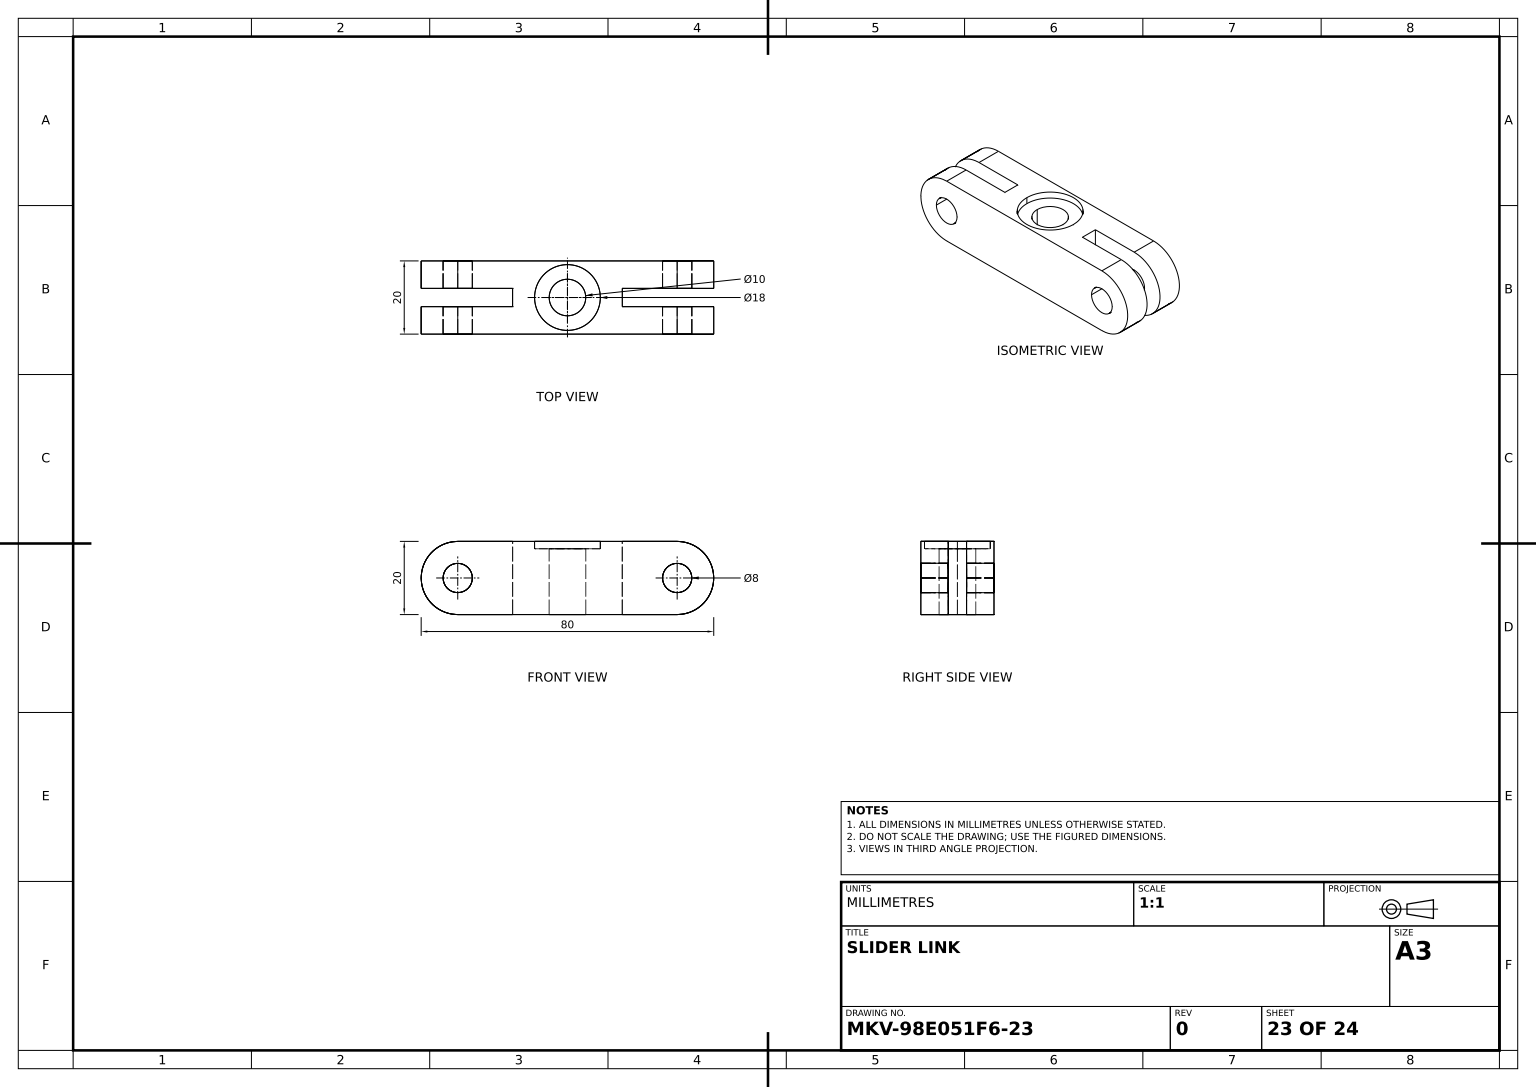
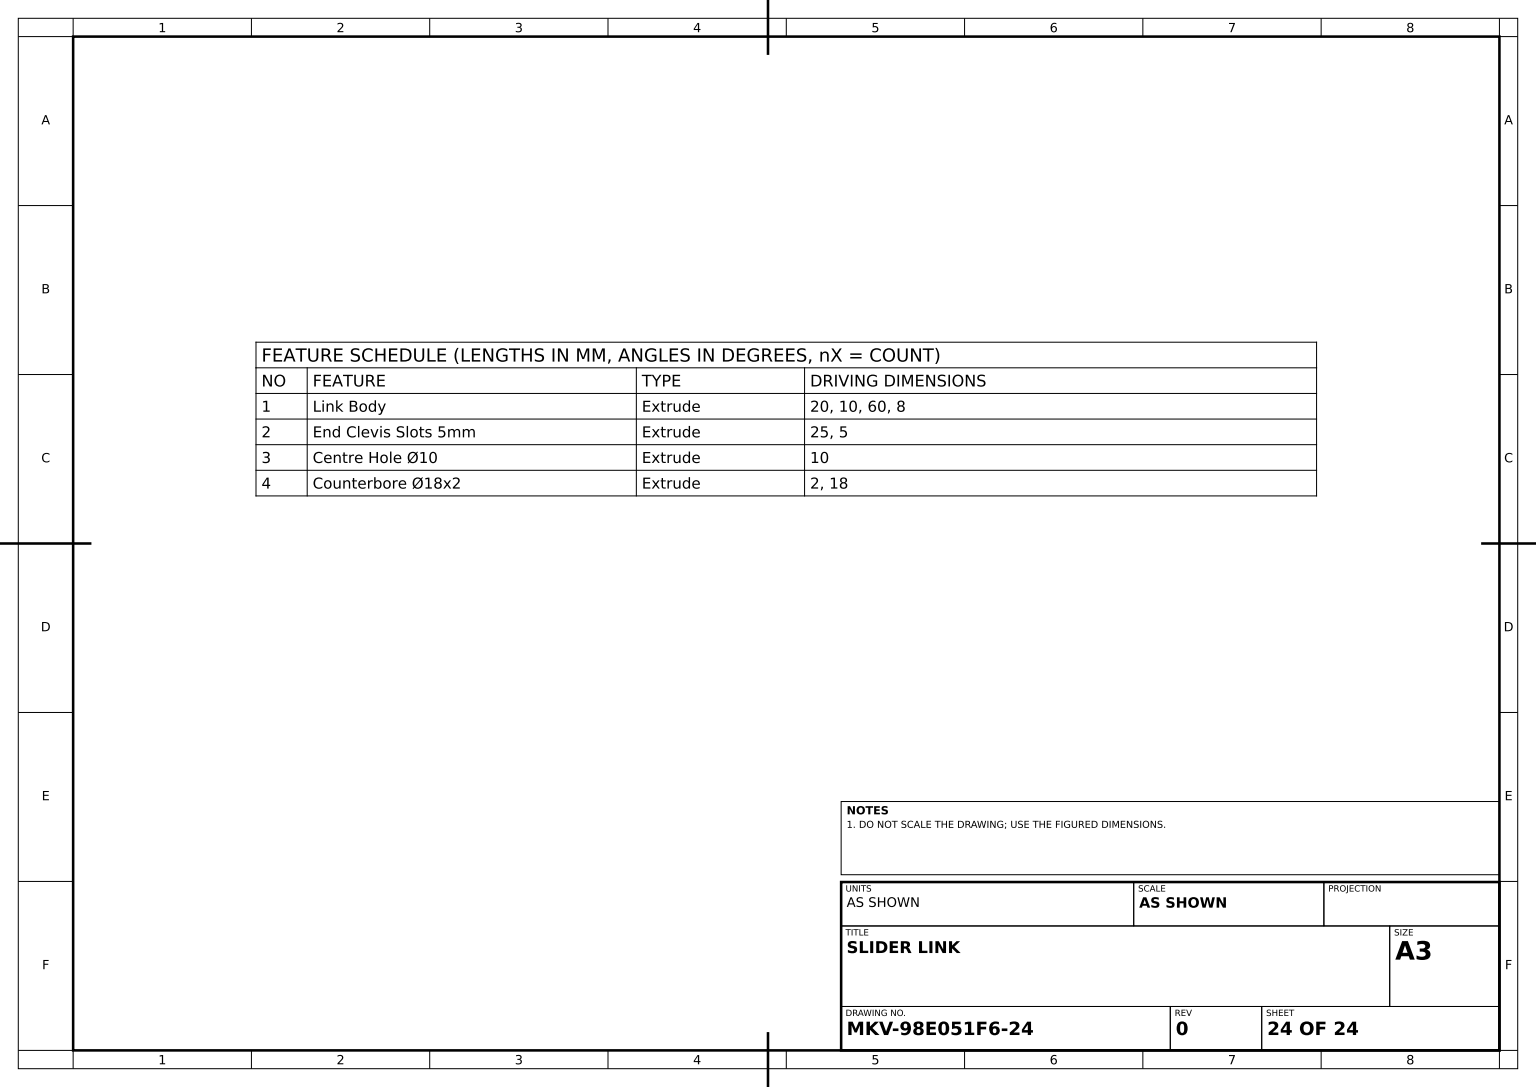
ISO-10303-21;
HEADER;
FILE_DESCRIPTION((''),'2;1');
FILE_NAME('','',(''),(''),'','','');
FILE_SCHEMA(('AUTOMOTIVE_DESIGN'));
ENDSEC;
DATA;
#1=APPLICATION_CONTEXT('');
#2=PRODUCT_CONTEXT('',#1,'mechanical');
#3=PRODUCT('','','',(#2));
#4=PRODUCT_DEFINITION_FORMATION('','',#3);
#5=PRODUCT_DEFINITION_CONTEXT('',#1,'design');
#6=PRODUCT_DEFINITION('','',#4,#5);
#7=PRODUCT_DEFINITION_SHAPE('','',#6);
#8=(LENGTH_UNIT()NAMED_UNIT(*)SI_UNIT(.MILLI.,.METRE.));
#9=(NAMED_UNIT(*)PLANE_ANGLE_UNIT()SI_UNIT($,.RADIAN.));
#10=(NAMED_UNIT(*)SI_UNIT($,.STERADIAN.)SOLID_ANGLE_UNIT());
#11=UNCERTAINTY_MEASURE_WITH_UNIT(LENGTH_MEASURE(1.E-05),#8,'distance_accuracy_value','');
#12=(GEOMETRIC_REPRESENTATION_CONTEXT(3)GLOBAL_UNCERTAINTY_ASSIGNED_CONTEXT((#11))GLOBAL_UNIT_ASSIGNED_CONTEXT((#8,#9,#10))REPRESENTATION_CONTEXT('',''));
#13=CARTESIAN_POINT('',(-30.,-10.,10.));
#14=VERTEX_POINT('',#13);
#15=CARTESIAN_POINT('',(-30.,-10.,2.5));
#16=VERTEX_POINT('',#15);
#17=DIRECTION('',(0.,0.,-1.));
#18=VECTOR('',#17,1000.);
#19=LINE('',#13,#18);
#20=EDGE_CURVE('',#14,#16,#19,.T.);
#21=ORIENTED_EDGE('',*,*,#20,.F.);
#22=CARTESIAN_POINT('',(-40.,0.,10.));
#23=VERTEX_POINT('',#22);
#24=CARTESIAN_POINT('',(-30.,0.,10.));
#25=DIRECTION('',(0.,0.,1.));
#26=DIRECTION('',(1.,0.,0.));
#27=AXIS2_PLACEMENT_3D('',#24,#25,#26);
#28=CIRCLE('',#27,10.);
#29=EDGE_CURVE('',#23,#14,#28,.T.);
#30=ORIENTED_EDGE('',*,*,#29,.F.);
#31=CARTESIAN_POINT('',(-40.,0.,2.5));
#32=VERTEX_POINT('',#31);
#33=LINE('',#22,#18);
#34=EDGE_CURVE('',#23,#32,#33,.T.);
#35=ORIENTED_EDGE('',*,*,#34,.T.);
#36=CARTESIAN_POINT('',(-30.,0.,2.5));
#37=AXIS2_PLACEMENT_3D('',#36,#25,#26);
#38=CIRCLE('',#37,10.);
#39=EDGE_CURVE('',#32,#16,#38,.T.);
#40=ORIENTED_EDGE('',*,*,#39,.T.);
#41=EDGE_LOOP('',(#21,#30,#35,#40));
#42=FACE_OUTER_BOUND('',#41,.T.);
#43=DIRECTION('',(-1.,0.,0.));
#44=AXIS2_PLACEMENT_3D('',#24,#17,#43);
#45=CYLINDRICAL_SURFACE('',#44,10.);
#46=ADVANCED_FACE('',(#42),#45,.T.);
#47=CARTESIAN_POINT('',(-34.,0.,10.));
#48=VERTEX_POINT('',#47);
#49=CARTESIAN_POINT('',(-26.,0.,10.));
#50=VERTEX_POINT('',#49);
#51=CIRCLE('',#27,4.);
#52=EDGE_CURVE('',#48,#50,#51,.T.);
#53=ORIENTED_EDGE('',*,*,#52,.T.);
#54=CARTESIAN_POINT('',(-26.,0.,2.5));
#55=VERTEX_POINT('',#54);
#56=LINE('',#49,#18);
#57=EDGE_CURVE('',#50,#55,#56,.T.);
#58=ORIENTED_EDGE('',*,*,#57,.T.);
#59=CARTESIAN_POINT('',(-34.,0.,2.5));
#60=VERTEX_POINT('',#59);
#61=CIRCLE('',#37,4.);
#62=EDGE_CURVE('',#60,#55,#61,.T.);
#63=ORIENTED_EDGE('',*,*,#62,.F.);
#64=LINE('',#47,#18);
#65=EDGE_CURVE('',#48,#60,#64,.T.);
#66=ORIENTED_EDGE('',*,*,#65,.F.);
#67=EDGE_LOOP('',(#53,#58,#63,#66));
#68=FACE_OUTER_BOUND('',#67,.T.);
#69=CYLINDRICAL_SURFACE('',#44,4.);
#70=ADVANCED_FACE('',(#68),#69,.F.);
#71=CARTESIAN_POINT('',(9.,8.,0.));
#72=VERTEX_POINT('',#71);
#73=CARTESIAN_POINT('',(-9.,8.,0.));
#74=VERTEX_POINT('',#73);
#75=CARTESIAN_POINT('',(0.,8.,0.));
#76=DIRECTION('',(0.,1.,0.));
#77=AXIS2_PLACEMENT_3D('',#75,#76,#43);
#78=CIRCLE('',#77,9.);
#79=EDGE_CURVE('',#72,#74,#78,.T.);
#80=ORIENTED_EDGE('',*,*,#79,.T.);
#81=EDGE_CURVE('',#74,#72,#78,.T.);
#82=ORIENTED_EDGE('',*,*,#81,.T.);
#83=EDGE_LOOP('',(#80,#82));
#84=FACE_OUTER_BOUND('',#83,.T.);
#85=CARTESIAN_POINT('',(5.,8.,0.));
#86=VERTEX_POINT('',#85);
#87=CARTESIAN_POINT('',(-5.,8.,0.));
#88=VERTEX_POINT('',#87);
#89=DIRECTION('',(0.,-1.,0.));
#90=AXIS2_PLACEMENT_3D('',#75,#89,#43);
#91=CIRCLE('',#90,5.);
#92=EDGE_CURVE('',#86,#88,#91,.T.);
#93=ORIENTED_EDGE('',*,*,#92,.T.);
#94=EDGE_CURVE('',#88,#86,#91,.T.);
#95=ORIENTED_EDGE('',*,*,#94,.T.);
#96=EDGE_LOOP('',(#93,#95));
#97=FACE_BOUND('',#96,.T.);
#98=PLANE('',#77);
#99=ADVANCED_FACE('',(#84,#97),#98,.T.);
#100=CARTESIAN_POINT('',(30.,-10.,-2.5));
#101=VERTEX_POINT('',#100);
#102=CARTESIAN_POINT('',(30.,-10.,-10.));
#103=VERTEX_POINT('',#102);
#104=CARTESIAN_POINT('',(30.,-10.,10.));
#105=LINE('',#104,#18);
#106=EDGE_CURVE('',#101,#103,#105,.T.);
#107=ORIENTED_EDGE('',*,*,#106,.T.);
#108=CARTESIAN_POINT('',(30.,10.,-10.));
#109=VERTEX_POINT('',#108);
#110=CARTESIAN_POINT('',(30.,0.,-10.));
#111=AXIS2_PLACEMENT_3D('',#110,#25,#26);
#112=CIRCLE('',#111,10.);
#113=EDGE_CURVE('',#103,#109,#112,.T.);
#114=ORIENTED_EDGE('',*,*,#113,.T.);
#115=CARTESIAN_POINT('',(30.,10.,-2.5));
#116=VERTEX_POINT('',#115);
#117=CARTESIAN_POINT('',(30.,10.,10.));
#118=LINE('',#117,#18);
#119=EDGE_CURVE('',#116,#109,#118,.T.);
#120=ORIENTED_EDGE('',*,*,#119,.F.);
#121=CARTESIAN_POINT('',(30.,0.,-2.5));
#122=AXIS2_PLACEMENT_3D('',#121,#17,#43);
#123=CIRCLE('',#122,10.);
#124=EDGE_CURVE('',#116,#101,#123,.T.);
#125=ORIENTED_EDGE('',*,*,#124,.T.);
#126=EDGE_LOOP('',(#107,#114,#120,#125));
#127=FACE_OUTER_BOUND('',#126,.T.);
#128=CARTESIAN_POINT('',(30.,0.,10.));
#129=AXIS2_PLACEMENT_3D('',#128,#17,#43);
#130=CYLINDRICAL_SURFACE('',#129,10.);
#131=ADVANCED_FACE('',(#127),#130,.T.);
#132=CARTESIAN_POINT('',(34.,0.,2.5));
#133=VERTEX_POINT('',#132);
#134=CARTESIAN_POINT('',(26.,0.,2.5));
#135=VERTEX_POINT('',#134);
#136=CARTESIAN_POINT('',(30.,0.,2.5));
#137=AXIS2_PLACEMENT_3D('',#136,#25,#26);
#138=CIRCLE('',#137,4.);
#139=EDGE_CURVE('',#133,#135,#138,.T.);
#140=ORIENTED_EDGE('',*,*,#139,.F.);
#141=CARTESIAN_POINT('',(34.,0.,10.));
#142=VERTEX_POINT('',#141);
#143=LINE('',#141,#18);
#144=EDGE_CURVE('',#142,#133,#143,.T.);
#145=ORIENTED_EDGE('',*,*,#144,.F.);
#146=CARTESIAN_POINT('',(26.,0.,10.));
#147=VERTEX_POINT('',#146);
#148=AXIS2_PLACEMENT_3D('',#128,#25,#26);
#149=CIRCLE('',#148,4.);
#150=EDGE_CURVE('',#142,#147,#149,.T.);
#151=ORIENTED_EDGE('',*,*,#150,.T.);
#152=LINE('',#146,#18);
#153=EDGE_CURVE('',#147,#135,#152,.T.);
#154=ORIENTED_EDGE('',*,*,#153,.T.);
#155=EDGE_LOOP('',(#140,#145,#151,#154));
#156=FACE_OUTER_BOUND('',#155,.T.);
#157=CYLINDRICAL_SURFACE('',#129,4.);
#158=ADVANCED_FACE('',(#156),#157,.F.);
#159=CARTESIAN_POINT('',(34.,0.,-2.5));
#160=VERTEX_POINT('',#159);
#161=CARTESIAN_POINT('',(34.,0.,-10.));
#162=VERTEX_POINT('',#161);
#163=EDGE_CURVE('',#160,#162,#143,.T.);
#164=ORIENTED_EDGE('',*,*,#163,.F.);
#165=CARTESIAN_POINT('',(26.,0.,-2.5));
#166=VERTEX_POINT('',#165);
#167=CIRCLE('',#122,4.);
#168=EDGE_CURVE('',#166,#160,#167,.T.);
#169=ORIENTED_EDGE('',*,*,#168,.F.);
#170=CARTESIAN_POINT('',(26.,0.,-10.));
#171=VERTEX_POINT('',#170);
#172=EDGE_CURVE('',#166,#171,#152,.T.);
#173=ORIENTED_EDGE('',*,*,#172,.T.);
#174=CIRCLE('',#111,4.);
#175=EDGE_CURVE('',#162,#171,#174,.T.);
#176=ORIENTED_EDGE('',*,*,#175,.F.);
#177=EDGE_LOOP('',(#164,#169,#173,#176));
#178=FACE_OUTER_BOUND('',#177,.T.);
#179=ADVANCED_FACE('',(#178),#157,.F.);
#180=EDGE_CURVE('',#50,#48,#51,.T.);
#181=ORIENTED_EDGE('',*,*,#180,.F.);
#182=ORIENTED_EDGE('',*,*,#52,.F.);
#183=EDGE_LOOP('',(#181,#182));
#184=FACE_BOUND('',#183,.T.);
#185=EDGE_CURVE('',#147,#142,#149,.T.);
#186=ORIENTED_EDGE('',*,*,#185,.F.);
#187=ORIENTED_EDGE('',*,*,#150,.F.);
#188=EDGE_LOOP('',(#186,#187));
#189=FACE_BOUND('',#188,.T.);
#190=ORIENTED_EDGE('',*,*,#29,.T.);
#191=VERTEX_POINT('',#104);
#192=VECTOR('',#26,1000.);
#193=LINE('',#13,#192);
#194=EDGE_CURVE('',#14,#191,#193,.T.);
#195=ORIENTED_EDGE('',*,*,#194,.T.);
#196=VERTEX_POINT('',#117);
#197=CIRCLE('',#148,10.);
#198=EDGE_CURVE('',#191,#196,#197,.T.);
#199=ORIENTED_EDGE('',*,*,#198,.T.);
#200=CARTESIAN_POINT('',(-30.,10.,10.));
#201=VERTEX_POINT('',#200);
#202=VECTOR('',#43,1000.);
#203=LINE('',#200,#202);
#204=EDGE_CURVE('',#196,#201,#203,.T.);
#205=ORIENTED_EDGE('',*,*,#204,.T.);
#206=EDGE_CURVE('',#201,#23,#28,.T.);
#207=ORIENTED_EDGE('',*,*,#206,.T.);
#208=EDGE_LOOP('',(#190,#195,#199,#205,#207));
#209=FACE_OUTER_BOUND('',#208,.T.);
#210=PLANE('',#27);
#211=ADVANCED_FACE('',(#184,#189,#209),#210,.T.);
#212=CARTESIAN_POINT('',(-15.,10.,2.5));
#213=VERTEX_POINT('',#212);
#214=CARTESIAN_POINT('',(-15.,10.,-2.5));
#215=VERTEX_POINT('',#214);
#216=LINE('',#212,#18);
#217=EDGE_CURVE('',#213,#215,#216,.T.);
#218=ORIENTED_EDGE('',*,*,#217,.T.);
#219=CARTESIAN_POINT('',(-15.,-10.,-2.5));
#220=VERTEX_POINT('',#219);
#221=VECTOR('',#76,1000.);
#222=LINE('',#219,#221);
#223=EDGE_CURVE('',#220,#215,#222,.T.);
#224=ORIENTED_EDGE('',*,*,#223,.F.);
#225=CARTESIAN_POINT('',(-15.,-10.,2.5));
#226=VERTEX_POINT('',#225);
#227=LINE('',#225,#18);
#228=EDGE_CURVE('',#226,#220,#227,.T.);
#229=ORIENTED_EDGE('',*,*,#228,.F.);
#230=LINE('',#225,#221);
#231=EDGE_CURVE('',#226,#213,#230,.T.);
#232=ORIENTED_EDGE('',*,*,#231,.T.);
#233=EDGE_LOOP('',(#218,#224,#229,#232));
#234=FACE_OUTER_BOUND('',#233,.T.);
#235=AXIS2_PLACEMENT_3D('',#225,#26,#76);
#236=PLANE('',#235);
#237=ADVANCED_FACE('',(#234),#236,.F.);
#238=CARTESIAN_POINT('',(9.,10.,0.));
#239=VERTEX_POINT('',#238);
#240=CARTESIAN_POINT('',(-9.,10.,0.));
#241=VERTEX_POINT('',#240);
#242=CARTESIAN_POINT('',(0.,10.,0.));
#243=AXIS2_PLACEMENT_3D('',#242,#76,#43);
#244=CIRCLE('',#243,9.);
#245=EDGE_CURVE('',#239,#241,#244,.T.);
#246=ORIENTED_EDGE('',*,*,#245,.T.);
#247=LINE('',#73,#221);
#248=EDGE_CURVE('',#74,#241,#247,.T.);
#249=ORIENTED_EDGE('',*,*,#248,.F.);
#250=ORIENTED_EDGE('',*,*,#79,.F.);
#251=LINE('',#71,#221);
#252=EDGE_CURVE('',#72,#239,#251,.T.);
#253=ORIENTED_EDGE('',*,*,#252,.T.);
#254=EDGE_LOOP('',(#246,#249,#250,#253));
#255=FACE_OUTER_BOUND('',#254,.T.);
#256=CYLINDRICAL_SURFACE('',#77,9.);
#257=ADVANCED_FACE('',(#255),#256,.F.);
#258=ORIENTED_EDGE('',*,*,#168,.T.);
#259=EDGE_CURVE('',#160,#166,#167,.T.);
#260=ORIENTED_EDGE('',*,*,#259,.T.);
#261=EDGE_LOOP('',(#258,#260));
#262=FACE_BOUND('',#261,.T.);
#263=CARTESIAN_POINT('',(15.,-10.,-2.5));
#264=VERTEX_POINT('',#263);
#265=LINE('',#263,#202);
#266=EDGE_CURVE('',#101,#264,#265,.T.);
#267=ORIENTED_EDGE('',*,*,#266,.F.);
#268=ORIENTED_EDGE('',*,*,#124,.F.);
#269=CARTESIAN_POINT('',(15.,10.,-2.5));
#270=VERTEX_POINT('',#269);
#271=LINE('',#269,#202);
#272=EDGE_CURVE('',#116,#270,#271,.T.);
#273=ORIENTED_EDGE('',*,*,#272,.T.);
#274=LINE('',#263,#221);
#275=EDGE_CURVE('',#264,#270,#274,.T.);
#276=ORIENTED_EDGE('',*,*,#275,.F.);
#277=EDGE_LOOP('',(#267,#268,#273,#276));
#278=FACE_OUTER_BOUND('',#277,.T.);
#279=AXIS2_PLACEMENT_3D('',#263,#17,#43);
#280=PLANE('',#279);
#281=ADVANCED_FACE('',(#262,#278),#280,.F.);
#282=CARTESIAN_POINT('',(-5.,-10.,0.));
#283=VERTEX_POINT('',#282);
#284=CARTESIAN_POINT('',(5.,-10.,0.));
#285=VERTEX_POINT('',#284);
#286=CARTESIAN_POINT('',(0.,-10.,0.));
#287=AXIS2_PLACEMENT_3D('',#286,#76,#43);
#288=CIRCLE('',#287,5.);
#289=EDGE_CURVE('',#283,#285,#288,.T.);
#290=ORIENTED_EDGE('',*,*,#289,.F.);
#291=LINE('',#282,#221);
#292=EDGE_CURVE('',#283,#88,#291,.T.);
#293=ORIENTED_EDGE('',*,*,#292,.T.);
#294=ORIENTED_EDGE('',*,*,#92,.F.);
#295=LINE('',#284,#221);
#296=EDGE_CURVE('',#285,#86,#295,.T.);
#297=ORIENTED_EDGE('',*,*,#296,.F.);
#298=EDGE_LOOP('',(#290,#293,#294,#297));
#299=FACE_OUTER_BOUND('',#298,.T.);
#300=CYLINDRICAL_SURFACE('',#287,5.);
#301=ADVANCED_FACE('',(#299),#300,.F.);
#302=CARTESIAN_POINT('',(-40.,0.,-2.5));
#303=VERTEX_POINT('',#302);
#304=CARTESIAN_POINT('',(-40.,0.,-10.));
#305=VERTEX_POINT('',#304);
#306=EDGE_CURVE('',#303,#305,#33,.T.);
#307=ORIENTED_EDGE('',*,*,#306,.F.);
#308=CARTESIAN_POINT('',(-30.,10.,-2.5));
#309=VERTEX_POINT('',#308);
#310=CARTESIAN_POINT('',(-30.,0.,-2.5));
#311=AXIS2_PLACEMENT_3D('',#310,#17,#43);
#312=CIRCLE('',#311,10.);
#313=EDGE_CURVE('',#303,#309,#312,.T.);
#314=ORIENTED_EDGE('',*,*,#313,.T.);
#315=CARTESIAN_POINT('',(-30.,10.,-10.));
#316=VERTEX_POINT('',#315);
#317=LINE('',#200,#18);
#318=EDGE_CURVE('',#309,#316,#317,.T.);
#319=ORIENTED_EDGE('',*,*,#318,.T.);
#320=CARTESIAN_POINT('',(-30.,0.,-10.));
#321=AXIS2_PLACEMENT_3D('',#320,#25,#26);
#322=CIRCLE('',#321,10.);
#323=EDGE_CURVE('',#316,#305,#322,.T.);
#324=ORIENTED_EDGE('',*,*,#323,.T.);
#325=EDGE_LOOP('',(#307,#314,#319,#324));
#326=FACE_OUTER_BOUND('',#325,.T.);
#327=ADVANCED_FACE('',(#326),#45,.T.);
#328=CARTESIAN_POINT('',(-34.,0.,-10.));
#329=VERTEX_POINT('',#328);
#330=CARTESIAN_POINT('',(-26.,0.,-10.));
#331=VERTEX_POINT('',#330);
#332=CIRCLE('',#321,4.);
#333=EDGE_CURVE('',#329,#331,#332,.T.);
#334=ORIENTED_EDGE('',*,*,#333,.F.);
#335=CARTESIAN_POINT('',(-34.,0.,-2.5));
#336=VERTEX_POINT('',#335);
#337=EDGE_CURVE('',#336,#329,#64,.T.);
#338=ORIENTED_EDGE('',*,*,#337,.F.);
#339=CARTESIAN_POINT('',(-26.,0.,-2.5));
#340=VERTEX_POINT('',#339);
#341=CIRCLE('',#311,4.);
#342=EDGE_CURVE('',#340,#336,#341,.T.);
#343=ORIENTED_EDGE('',*,*,#342,.F.);
#344=EDGE_CURVE('',#340,#331,#56,.T.);
#345=ORIENTED_EDGE('',*,*,#344,.T.);
#346=EDGE_LOOP('',(#334,#338,#343,#345));
#347=FACE_OUTER_BOUND('',#346,.T.);
#348=ADVANCED_FACE('',(#347),#69,.F.);
#349=ORIENTED_EDGE('',*,*,#333,.T.);
#350=EDGE_CURVE('',#331,#329,#332,.T.);
#351=ORIENTED_EDGE('',*,*,#350,.T.);
#352=EDGE_LOOP('',(#349,#351));
#353=FACE_BOUND('',#352,.T.);
#354=LINE('',#315,#202);
#355=EDGE_CURVE('',#109,#316,#354,.T.);
#356=ORIENTED_EDGE('',*,*,#355,.F.);
#357=ORIENTED_EDGE('',*,*,#113,.F.);
#358=CARTESIAN_POINT('',(-30.,-10.,-10.));
#359=VERTEX_POINT('',#358);
#360=LINE('',#358,#192);
#361=EDGE_CURVE('',#359,#103,#360,.T.);
#362=ORIENTED_EDGE('',*,*,#361,.F.);
#363=EDGE_CURVE('',#305,#359,#322,.T.);
#364=ORIENTED_EDGE('',*,*,#363,.F.);
#365=ORIENTED_EDGE('',*,*,#323,.F.);
#366=EDGE_LOOP('',(#356,#357,#362,#364,#365));
#367=FACE_OUTER_BOUND('',#366,.T.);
#368=ORIENTED_EDGE('',*,*,#175,.T.);
#369=EDGE_CURVE('',#171,#162,#174,.T.);
#370=ORIENTED_EDGE('',*,*,#369,.T.);
#371=EDGE_LOOP('',(#368,#370));
#372=FACE_BOUND('',#371,.T.);
#373=PLANE('',#321);
#374=ADVANCED_FACE('',(#353,#367,#372),#373,.F.);
#375=ORIENTED_EDGE('',*,*,#180,.T.);
#376=ORIENTED_EDGE('',*,*,#65,.T.);
#377=EDGE_CURVE('',#55,#60,#61,.T.);
#378=ORIENTED_EDGE('',*,*,#377,.F.);
#379=ORIENTED_EDGE('',*,*,#57,.F.);
#380=EDGE_LOOP('',(#375,#376,#378,#379));
#381=FACE_OUTER_BOUND('',#380,.T.);
#382=ADVANCED_FACE('',(#381),#69,.F.);
#383=ORIENTED_EDGE('',*,*,#313,.F.);
#384=CARTESIAN_POINT('',(-30.,-10.,-2.5));
#385=VERTEX_POINT('',#384);
#386=EDGE_CURVE('',#385,#303,#312,.T.);
#387=ORIENTED_EDGE('',*,*,#386,.F.);
#388=LINE('',#219,#202);
#389=EDGE_CURVE('',#220,#385,#388,.T.);
#390=ORIENTED_EDGE('',*,*,#389,.F.);
#391=ORIENTED_EDGE('',*,*,#223,.T.);
#392=LINE('',#214,#202);
#393=EDGE_CURVE('',#215,#309,#392,.T.);
#394=ORIENTED_EDGE('',*,*,#393,.T.);
#395=EDGE_LOOP('',(#383,#387,#390,#391,#394));
#396=FACE_OUTER_BOUND('',#395,.T.);
#397=EDGE_CURVE('',#336,#340,#341,.T.);
#398=ORIENTED_EDGE('',*,*,#397,.T.);
#399=ORIENTED_EDGE('',*,*,#342,.T.);
#400=EDGE_LOOP('',(#398,#399));
#401=FACE_BOUND('',#400,.T.);
#402=AXIS2_PLACEMENT_3D('',#219,#17,#43);
#403=PLANE('',#402);
#404=ADVANCED_FACE('',(#396,#401),#403,.F.);
#405=CARTESIAN_POINT('',(30.,-10.,2.5));
#406=VERTEX_POINT('',#405);
#407=EDGE_CURVE('',#191,#406,#105,.T.);
#408=ORIENTED_EDGE('',*,*,#407,.T.);
#409=CARTESIAN_POINT('',(30.,10.,2.5));
#410=VERTEX_POINT('',#409);
#411=CIRCLE('',#137,10.);
#412=EDGE_CURVE('',#406,#410,#411,.T.);
#413=ORIENTED_EDGE('',*,*,#412,.T.);
#414=EDGE_CURVE('',#196,#410,#118,.T.);
#415=ORIENTED_EDGE('',*,*,#414,.F.);
#416=ORIENTED_EDGE('',*,*,#198,.F.);
#417=EDGE_LOOP('',(#408,#413,#415,#416));
#418=FACE_OUTER_BOUND('',#417,.T.);
#419=ADVANCED_FACE('',(#418),#130,.T.);
#420=EDGE_CURVE('',#135,#133,#138,.T.);
#421=ORIENTED_EDGE('',*,*,#420,.F.);
#422=ORIENTED_EDGE('',*,*,#153,.F.);
#423=ORIENTED_EDGE('',*,*,#185,.T.);
#424=ORIENTED_EDGE('',*,*,#144,.T.);
#425=EDGE_LOOP('',(#421,#422,#423,#424));
#426=FACE_OUTER_BOUND('',#425,.T.);
#427=ADVANCED_FACE('',(#426),#157,.F.);
#428=ORIENTED_EDGE('',*,*,#420,.T.);
#429=ORIENTED_EDGE('',*,*,#139,.T.);
#430=EDGE_LOOP('',(#428,#429));
#431=FACE_BOUND('',#430,.T.);
#432=ORIENTED_EDGE('',*,*,#412,.F.);
#433=CARTESIAN_POINT('',(15.,-10.,2.5));
#434=VERTEX_POINT('',#433);
#435=LINE('',#433,#192);
#436=EDGE_CURVE('',#434,#406,#435,.T.);
#437=ORIENTED_EDGE('',*,*,#436,.F.);
#438=CARTESIAN_POINT('',(15.,10.,2.5));
#439=VERTEX_POINT('',#438);
#440=LINE('',#433,#221);
#441=EDGE_CURVE('',#434,#439,#440,.T.);
#442=ORIENTED_EDGE('',*,*,#441,.T.);
#443=LINE('',#438,#192);
#444=EDGE_CURVE('',#439,#410,#443,.T.);
#445=ORIENTED_EDGE('',*,*,#444,.T.);
#446=EDGE_LOOP('',(#432,#437,#442,#445));
#447=FACE_OUTER_BOUND('',#446,.T.);
#448=AXIS2_PLACEMENT_3D('',#433,#25,#26);
#449=PLANE('',#448);
#450=ADVANCED_FACE('',(#431,#447),#449,.F.);
#451=ORIENTED_EDGE('',*,*,#248,.T.);
#452=EDGE_CURVE('',#241,#239,#244,.T.);
#453=ORIENTED_EDGE('',*,*,#452,.T.);
#454=ORIENTED_EDGE('',*,*,#252,.F.);
#455=ORIENTED_EDGE('',*,*,#81,.F.);
#456=EDGE_LOOP('',(#451,#453,#454,#455));
#457=FACE_OUTER_BOUND('',#456,.T.);
#458=ADVANCED_FACE('',(#457),#256,.F.);
#459=LINE('',#225,#192);
#460=EDGE_CURVE('',#16,#226,#459,.T.);
#461=ORIENTED_EDGE('',*,*,#460,.T.);
#462=ORIENTED_EDGE('',*,*,#228,.T.);
#463=ORIENTED_EDGE('',*,*,#389,.T.);
#464=EDGE_CURVE('',#385,#359,#19,.T.);
#465=ORIENTED_EDGE('',*,*,#464,.T.);
#466=ORIENTED_EDGE('',*,*,#361,.T.);
#467=ORIENTED_EDGE('',*,*,#106,.F.);
#468=ORIENTED_EDGE('',*,*,#266,.T.);
#469=VECTOR('',#25,1000.);
#470=LINE('',#433,#469);
#471=EDGE_CURVE('',#264,#434,#470,.T.);
#472=ORIENTED_EDGE('',*,*,#471,.T.);
#473=ORIENTED_EDGE('',*,*,#436,.T.);
#474=ORIENTED_EDGE('',*,*,#407,.F.);
#475=ORIENTED_EDGE('',*,*,#194,.F.);
#476=ORIENTED_EDGE('',*,*,#20,.T.);
#477=EDGE_LOOP('',(#461,#462,#463,#465,#466,#467,#468,#472,#473,#474,#475,#476));
#478=FACE_OUTER_BOUND('',#477,.T.);
#479=ORIENTED_EDGE('',*,*,#289,.T.);
#480=EDGE_CURVE('',#285,#283,#288,.T.);
#481=ORIENTED_EDGE('',*,*,#480,.T.);
#482=EDGE_LOOP('',(#479,#481));
#483=FACE_BOUND('',#482,.T.);
#484=AXIS2_PLACEMENT_3D('',#13,#76,#43);
#485=PLANE('',#484);
#486=ADVANCED_FACE('',(#478,#483),#485,.F.);
#487=ORIENTED_EDGE('',*,*,#296,.T.);
#488=ORIENTED_EDGE('',*,*,#94,.F.);
#489=ORIENTED_EDGE('',*,*,#292,.F.);
#490=ORIENTED_EDGE('',*,*,#480,.F.);
#491=EDGE_LOOP('',(#487,#488,#489,#490));
#492=FACE_OUTER_BOUND('',#491,.T.);
#493=ADVANCED_FACE('',(#492),#300,.F.);
#494=ORIENTED_EDGE('',*,*,#377,.T.);
#495=ORIENTED_EDGE('',*,*,#62,.T.);
#496=EDGE_LOOP('',(#494,#495));
#497=FACE_BOUND('',#496,.T.);
#498=ORIENTED_EDGE('',*,*,#231,.F.);
#499=ORIENTED_EDGE('',*,*,#460,.F.);
#500=ORIENTED_EDGE('',*,*,#39,.F.);
#501=CARTESIAN_POINT('',(-30.,10.,2.5));
#502=VERTEX_POINT('',#501);
#503=EDGE_CURVE('',#502,#32,#38,.T.);
#504=ORIENTED_EDGE('',*,*,#503,.F.);
#505=LINE('',#212,#192);
#506=EDGE_CURVE('',#502,#213,#505,.T.);
#507=ORIENTED_EDGE('',*,*,#506,.T.);
#508=EDGE_LOOP('',(#498,#499,#500,#504,#507));
#509=FACE_OUTER_BOUND('',#508,.T.);
#510=AXIS2_PLACEMENT_3D('',#225,#25,#26);
#511=PLANE('',#510);
#512=ADVANCED_FACE('',(#497,#509),#511,.F.);
#513=ORIENTED_EDGE('',*,*,#245,.F.);
#514=ORIENTED_EDGE('',*,*,#452,.F.);
#515=EDGE_LOOP('',(#513,#514));
#516=FACE_BOUND('',#515,.T.);
#517=EDGE_CURVE('',#201,#502,#317,.T.);
#518=ORIENTED_EDGE('',*,*,#517,.F.);
#519=ORIENTED_EDGE('',*,*,#204,.F.);
#520=ORIENTED_EDGE('',*,*,#414,.T.);
#521=ORIENTED_EDGE('',*,*,#444,.F.);
#522=LINE('',#438,#469);
#523=EDGE_CURVE('',#270,#439,#522,.T.);
#524=ORIENTED_EDGE('',*,*,#523,.F.);
#525=ORIENTED_EDGE('',*,*,#272,.F.);
#526=ORIENTED_EDGE('',*,*,#119,.T.);
#527=ORIENTED_EDGE('',*,*,#355,.T.);
#528=ORIENTED_EDGE('',*,*,#318,.F.);
#529=ORIENTED_EDGE('',*,*,#393,.F.);
#530=ORIENTED_EDGE('',*,*,#217,.F.);
#531=ORIENTED_EDGE('',*,*,#506,.F.);
#532=EDGE_LOOP('',(#518,#519,#520,#521,#524,#525,#526,#527,#528,#529,#530,#531));
#533=FACE_OUTER_BOUND('',#532,.T.);
#534=AXIS2_PLACEMENT_3D('',#200,#89,#26);
#535=PLANE('',#534);
#536=ADVANCED_FACE('',(#516,#533),#535,.F.);
#537=ORIENTED_EDGE('',*,*,#386,.T.);
#538=ORIENTED_EDGE('',*,*,#306,.T.);
#539=ORIENTED_EDGE('',*,*,#363,.T.);
#540=ORIENTED_EDGE('',*,*,#464,.F.);
#541=EDGE_LOOP('',(#537,#538,#539,#540));
#542=FACE_OUTER_BOUND('',#541,.T.);
#543=ADVANCED_FACE('',(#542),#45,.T.);
#544=ORIENTED_EDGE('',*,*,#163,.T.);
#545=ORIENTED_EDGE('',*,*,#369,.F.);
#546=ORIENTED_EDGE('',*,*,#172,.F.);
#547=ORIENTED_EDGE('',*,*,#259,.F.);
#548=EDGE_LOOP('',(#544,#545,#546,#547));
#549=FACE_OUTER_BOUND('',#548,.T.);
#550=ADVANCED_FACE('',(#549),#157,.F.);
#551=ORIENTED_EDGE('',*,*,#503,.T.);
#552=ORIENTED_EDGE('',*,*,#34,.F.);
#553=ORIENTED_EDGE('',*,*,#206,.F.);
#554=ORIENTED_EDGE('',*,*,#517,.T.);
#555=EDGE_LOOP('',(#551,#552,#553,#554));
#556=FACE_OUTER_BOUND('',#555,.T.);
#557=ADVANCED_FACE('',(#556),#45,.T.);
#558=ORIENTED_EDGE('',*,*,#471,.F.);
#559=ORIENTED_EDGE('',*,*,#275,.T.);
#560=ORIENTED_EDGE('',*,*,#523,.T.);
#561=ORIENTED_EDGE('',*,*,#441,.F.);
#562=EDGE_LOOP('',(#558,#559,#560,#561));
#563=FACE_OUTER_BOUND('',#562,.T.);
#564=AXIS2_PLACEMENT_3D('',#433,#43,#89);
#565=PLANE('',#564);
#566=ADVANCED_FACE('',(#563),#565,.F.);
#567=ORIENTED_EDGE('',*,*,#397,.F.);
#568=ORIENTED_EDGE('',*,*,#337,.T.);
#569=ORIENTED_EDGE('',*,*,#350,.F.);
#570=ORIENTED_EDGE('',*,*,#344,.F.);
#571=EDGE_LOOP('',(#567,#568,#569,#570));
#572=FACE_OUTER_BOUND('',#571,.T.);
#573=ADVANCED_FACE('',(#572),#69,.F.);
#574=CLOSED_SHELL('',(#46,#70,#99,#131,#158,#179,#211,#237,#257,#281,#301,#327,#348,#374,#382,#404,#419,#427,#450,#458,#486,#493,#512,#536,#543,#550,#557,#566,#573));
#575=MANIFOLD_SOLID_BREP('',#574);
#576=ADVANCED_BREP_SHAPE_REPRESENTATION('',(#575),#12);
#577=SHAPE_DEFINITION_REPRESENTATION(#7,#576);
ENDSEC;
END-ISO-10303-21;
